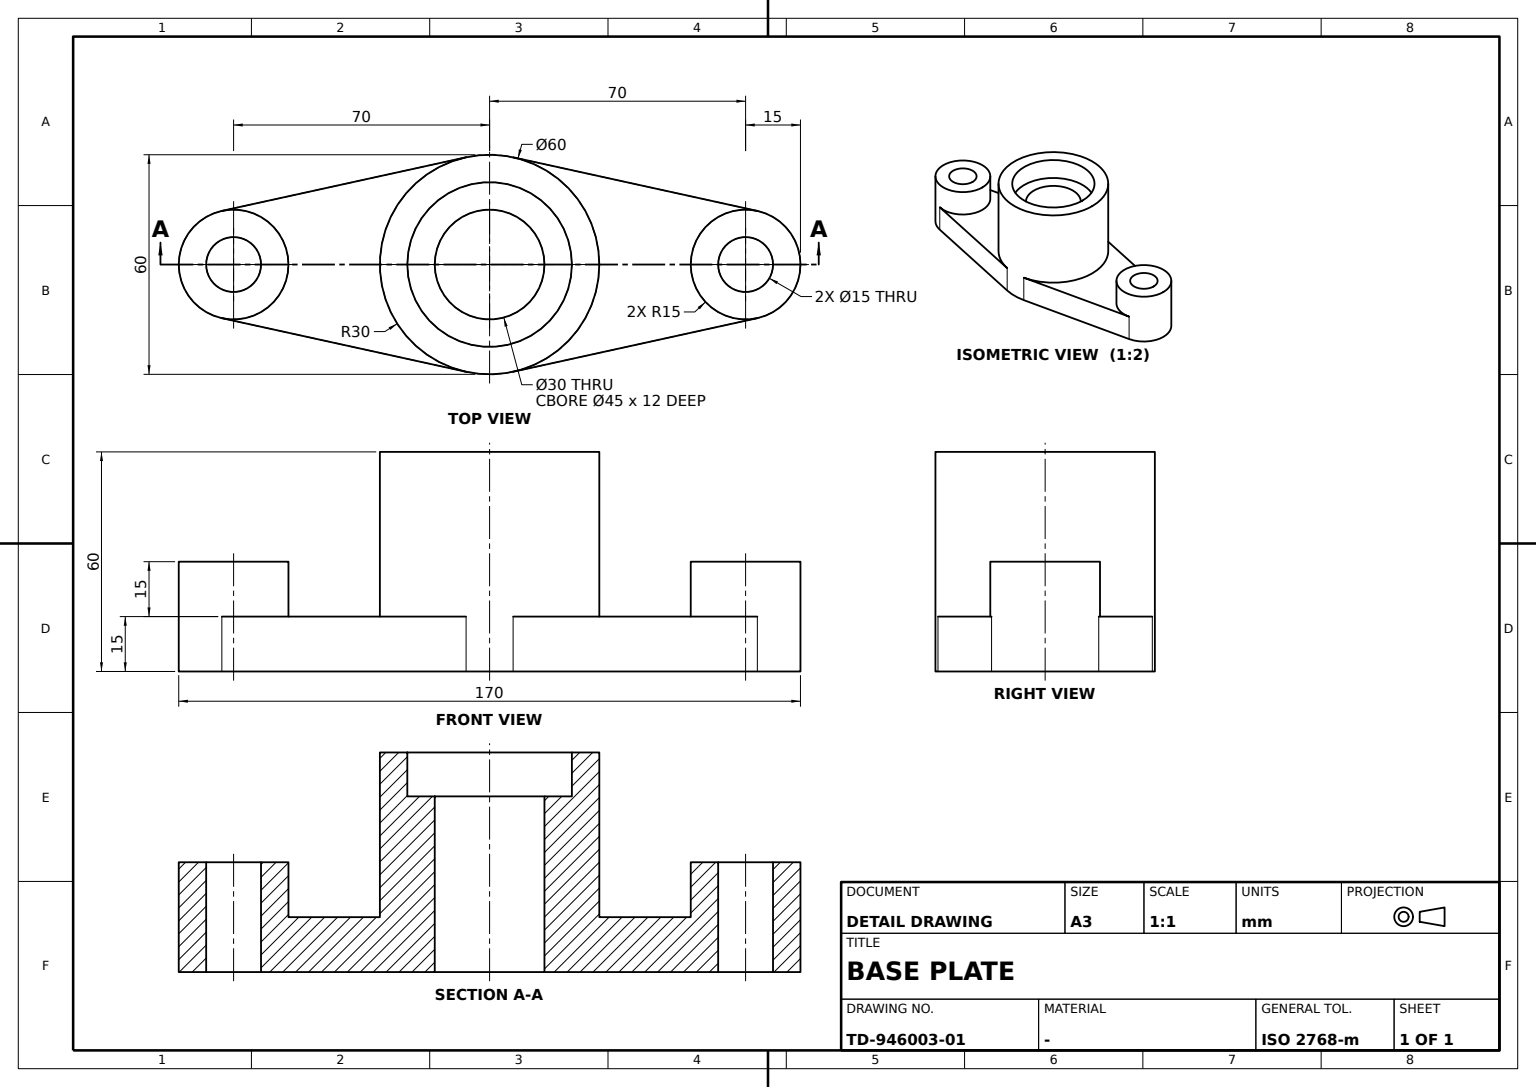
ISO-10303-21;
HEADER;
FILE_DESCRIPTION((''),'2;1');
FILE_NAME('','',(''),(''),'','','');
FILE_SCHEMA(('AUTOMOTIVE_DESIGN'));
ENDSEC;
DATA;
#1=APPLICATION_CONTEXT('');
#2=PRODUCT_CONTEXT('',#1,'mechanical');
#3=PRODUCT('','','',(#2));
#4=PRODUCT_DEFINITION_FORMATION('','',#3);
#5=PRODUCT_DEFINITION_CONTEXT('',#1,'design');
#6=PRODUCT_DEFINITION('','',#4,#5);
#7=PRODUCT_DEFINITION_SHAPE('','',#6);
#8=(LENGTH_UNIT()NAMED_UNIT(*)SI_UNIT(.MILLI.,.METRE.));
#9=(NAMED_UNIT(*)PLANE_ANGLE_UNIT()SI_UNIT($,.RADIAN.));
#10=(NAMED_UNIT(*)SI_UNIT($,.STERADIAN.)SOLID_ANGLE_UNIT());
#11=UNCERTAINTY_MEASURE_WITH_UNIT(LENGTH_MEASURE(0.005),#8,'distance_accuracy_value','');
#12=(GEOMETRIC_REPRESENTATION_CONTEXT(3)GLOBAL_UNCERTAINTY_ASSIGNED_CONTEXT((#11))GLOBAL_UNIT_ASSIGNED_CONTEXT((#8,#9,#10))REPRESENTATION_CONTEXT('',''));
#13=CARTESIAN_POINT('',(73.214286,14.651565,0.));
#14=VERTEX_POINT('',#13);
#15=CARTESIAN_POINT('',(73.214286,14.651565,15.));
#16=VERTEX_POINT('',#15);
#17=DIRECTION('',(0.,0.,1.));
#18=VECTOR('',#17,1000.);
#19=LINE('',#15,#18);
#20=EDGE_CURVE('',#14,#16,#19,.T.);
#21=ORIENTED_EDGE('',*,*,#20,.T.);
#22=CARTESIAN_POINT('',(73.214286,-14.651565,15.));
#23=VERTEX_POINT('',#22);
#24=CARTESIAN_POINT('',(70.,0.,15.));
#25=DIRECTION('',(1.,0.,0.));
#26=AXIS2_PLACEMENT_3D('',#24,#17,#25);
#27=CIRCLE('',#26,15.);
#28=EDGE_CURVE('',#16,#23,#27,.T.);
#29=ORIENTED_EDGE('',*,*,#28,.T.);
#30=CARTESIAN_POINT('',(73.214286,-14.651565,0.));
#31=VERTEX_POINT('',#30);
#32=LINE('',#22,#18);
#33=EDGE_CURVE('',#31,#23,#32,.T.);
#34=ORIENTED_EDGE('',*,*,#33,.F.);
#35=CARTESIAN_POINT('',(70.,0.,0.));
#36=AXIS2_PLACEMENT_3D('',#35,#17,#25);
#37=CIRCLE('',#36,15.);
#38=EDGE_CURVE('',#31,#14,#37,.T.);
#39=ORIENTED_EDGE('',*,*,#38,.T.);
#40=EDGE_LOOP('',(#21,#29,#34,#39));
#41=FACE_BOUND('',#40,.T.);
#42=CARTESIAN_POINT('',(85.,0.,30.));
#43=VERTEX_POINT('',#42);
#44=CARTESIAN_POINT('',(70.,0.,30.));
#45=AXIS2_PLACEMENT_3D('',#44,#17,#25);
#46=CIRCLE('',#45,15.);
#47=EDGE_CURVE('',#43,#43,#46,.T.);
#48=ORIENTED_EDGE('',*,*,#47,.F.);
#49=EDGE_LOOP('',(#48));
#50=FACE_BOUND('',#49,.T.);
#51=CYLINDRICAL_SURFACE('',#26,15.);
#52=ADVANCED_FACE('',(#41,#50),#51,.T.);
#53=CARTESIAN_POINT('',(-73.214286,-14.651565,15.));
#54=VERTEX_POINT('',#53);
#55=CARTESIAN_POINT('',(-6.428571,-29.303131,15.));
#56=VERTEX_POINT('',#55);
#57=DIRECTION('',(0.976771024,-0.214285714,0.));
#58=VECTOR('',#57,1000.);
#59=LINE('',#55,#58);
#60=EDGE_CURVE('',#54,#56,#59,.T.);
#61=ORIENTED_EDGE('',*,*,#60,.F.);
#62=CARTESIAN_POINT('',(-73.214286,-14.651565,0.));
#63=VERTEX_POINT('',#62);
#64=LINE('',#53,#18);
#65=EDGE_CURVE('',#63,#54,#64,.T.);
#66=ORIENTED_EDGE('',*,*,#65,.F.);
#67=CARTESIAN_POINT('',(-6.428571,-29.303131,0.));
#68=VERTEX_POINT('',#67);
#69=LINE('',#67,#58);
#70=EDGE_CURVE('',#63,#68,#69,.T.);
#71=ORIENTED_EDGE('',*,*,#70,.T.);
#72=CARTESIAN_POINT('',(-6.428571,-29.303131,30.));
#73=LINE('',#72,#18);
#74=EDGE_CURVE('',#68,#56,#73,.T.);
#75=ORIENTED_EDGE('',*,*,#74,.T.);
#76=EDGE_LOOP('',(#61,#66,#71,#75));
#77=FACE_BOUND('',#76,.T.);
#78=DIRECTION('',(-0.214285714,-0.976771024,0.));
#79=AXIS2_PLACEMENT_3D('',#62,#78,#57);
#80=PLANE('',#79);
#81=ADVANCED_FACE('',(#77),#80,.T.);
#82=CARTESIAN_POINT('',(22.5,0.,60.));
#83=VERTEX_POINT('',#82);
#84=CARTESIAN_POINT('',(0.,0.,60.));
#85=AXIS2_PLACEMENT_3D('',#84,#17,#25);
#86=CIRCLE('',#85,22.5);
#87=EDGE_CURVE('',#83,#83,#86,.T.);
#88=ORIENTED_EDGE('',*,*,#87,.F.);
#89=EDGE_LOOP('',(#88));
#90=FACE_BOUND('',#89,.T.);
#91=CARTESIAN_POINT('',(30.,0.,60.));
#92=VERTEX_POINT('',#91);
#93=CIRCLE('',#85,30.);
#94=EDGE_CURVE('',#92,#92,#93,.T.);
#95=ORIENTED_EDGE('',*,*,#94,.T.);
#96=EDGE_LOOP('',(#95));
#97=FACE_BOUND('',#96,.T.);
#98=PLANE('',#85);
#99=ADVANCED_FACE('',(#90,#97),#98,.T.);
#100=CARTESIAN_POINT('',(-73.214286,14.651565,15.));
#101=VERTEX_POINT('',#100);
#102=CARTESIAN_POINT('',(-6.428571,29.303131,15.));
#103=VERTEX_POINT('',#102);
#104=DIRECTION('',(0.976771024,0.214285714,0.));
#105=VECTOR('',#104,1000.);
#106=LINE('',#102,#105);
#107=EDGE_CURVE('',#101,#103,#106,.T.);
#108=ORIENTED_EDGE('',*,*,#107,.F.);
#109=CARTESIAN_POINT('',(-70.,0.,15.));
#110=AXIS2_PLACEMENT_3D('',#109,#17,#25);
#111=CIRCLE('',#110,15.);
#112=EDGE_CURVE('',#54,#101,#111,.T.);
#113=ORIENTED_EDGE('',*,*,#112,.F.);
#114=ORIENTED_EDGE('',*,*,#60,.T.);
#115=CARTESIAN_POINT('',(0.,0.,15.));
#116=AXIS2_PLACEMENT_3D('',#115,#17,#25);
#117=CIRCLE('',#116,30.);
#118=EDGE_CURVE('',#103,#56,#117,.T.);
#119=ORIENTED_EDGE('',*,*,#118,.F.);
#120=EDGE_LOOP('',(#108,#113,#114,#119));
#121=FACE_BOUND('',#120,.T.);
#122=PLANE('',#116);
#123=ADVANCED_FACE('',(#121),#122,.T.);
#124=ORIENTED_EDGE('',*,*,#87,.T.);
#125=EDGE_LOOP('',(#124));
#126=FACE_BOUND('',#125,.T.);
#127=CARTESIAN_POINT('',(22.5,0.,48.));
#128=VERTEX_POINT('',#127);
#129=CARTESIAN_POINT('',(0.,0.,48.));
#130=AXIS2_PLACEMENT_3D('',#129,#17,#25);
#131=CIRCLE('',#130,22.5);
#132=EDGE_CURVE('',#128,#128,#131,.T.);
#133=ORIENTED_EDGE('',*,*,#132,.F.);
#134=EDGE_LOOP('',(#133));
#135=FACE_BOUND('',#134,.T.);
#136=CARTESIAN_POINT('',(0.,0.,54.));
#137=AXIS2_PLACEMENT_3D('',#136,#17,#25);
#138=CYLINDRICAL_SURFACE('',#137,22.5);
#139=ADVANCED_FACE('',(#126,#135),#138,.F.);
#140=CARTESIAN_POINT('',(6.428571,29.303131,0.));
#141=VERTEX_POINT('',#140);
#142=CARTESIAN_POINT('',(6.428571,29.303131,15.));
#143=VERTEX_POINT('',#142);
#144=CARTESIAN_POINT('',(6.428571,29.303131,30.));
#145=LINE('',#144,#18);
#146=EDGE_CURVE('',#141,#143,#145,.T.);
#147=ORIENTED_EDGE('',*,*,#146,.T.);
#148=LINE('',#142,#58);
#149=EDGE_CURVE('',#143,#16,#148,.T.);
#150=ORIENTED_EDGE('',*,*,#149,.T.);
#151=ORIENTED_EDGE('',*,*,#20,.F.);
#152=LINE('',#140,#58);
#153=EDGE_CURVE('',#141,#14,#152,.T.);
#154=ORIENTED_EDGE('',*,*,#153,.F.);
#155=EDGE_LOOP('',(#147,#150,#151,#154));
#156=FACE_BOUND('',#155,.T.);
#157=AXIS2_PLACEMENT_3D('',#140,#78,#57);
#158=PLANE('',#157);
#159=ADVANCED_FACE('',(#156),#158,.F.);
#160=CARTESIAN_POINT('',(-62.5,0.,30.));
#161=VERTEX_POINT('',#160);
#162=CARTESIAN_POINT('',(-70.,0.,30.));
#163=AXIS2_PLACEMENT_3D('',#162,#17,#25);
#164=CIRCLE('',#163,7.5);
#165=EDGE_CURVE('',#161,#161,#164,.T.);
#166=ORIENTED_EDGE('',*,*,#165,.T.);
#167=EDGE_LOOP('',(#166));
#168=FACE_BOUND('',#167,.T.);
#169=CARTESIAN_POINT('',(-62.5,0.,0.));
#170=VERTEX_POINT('',#169);
#171=CARTESIAN_POINT('',(-70.,0.,0.));
#172=AXIS2_PLACEMENT_3D('',#171,#17,#25);
#173=CIRCLE('',#172,7.5);
#174=EDGE_CURVE('',#170,#170,#173,.T.);
#175=ORIENTED_EDGE('',*,*,#174,.F.);
#176=EDGE_LOOP('',(#175));
#177=FACE_BOUND('',#176,.T.);
#178=CYLINDRICAL_SURFACE('',#163,7.5);
#179=ADVANCED_FACE('',(#168,#177),#178,.F.);
#180=ORIENTED_EDGE('',*,*,#132,.T.);
#181=EDGE_LOOP('',(#180));
#182=FACE_BOUND('',#181,.T.);
#183=CARTESIAN_POINT('',(15.,0.,48.));
#184=VERTEX_POINT('',#183);
#185=CIRCLE('',#130,15.);
#186=EDGE_CURVE('',#184,#184,#185,.T.);
#187=ORIENTED_EDGE('',*,*,#186,.F.);
#188=EDGE_LOOP('',(#187));
#189=FACE_BOUND('',#188,.T.);
#190=PLANE('',#130);
#191=ADVANCED_FACE('',(#182,#189),#190,.T.);
#192=ORIENTED_EDGE('',*,*,#38,.F.);
#193=CARTESIAN_POINT('',(6.428571,-29.303131,0.));
#194=VERTEX_POINT('',#193);
#195=LINE('',#193,#105);
#196=EDGE_CURVE('',#194,#31,#195,.T.);
#197=ORIENTED_EDGE('',*,*,#196,.F.);
#198=CARTESIAN_POINT('',(0.,0.,0.));
#199=AXIS2_PLACEMENT_3D('',#198,#17,#25);
#200=CIRCLE('',#199,30.);
#201=EDGE_CURVE('',#68,#194,#200,.T.);
#202=ORIENTED_EDGE('',*,*,#201,.F.);
#203=ORIENTED_EDGE('',*,*,#70,.F.);
#204=CARTESIAN_POINT('',(-73.214286,14.651565,0.));
#205=VERTEX_POINT('',#204);
#206=CIRCLE('',#172,15.);
#207=EDGE_CURVE('',#205,#63,#206,.T.);
#208=ORIENTED_EDGE('',*,*,#207,.F.);
#209=CARTESIAN_POINT('',(-6.428571,29.303131,0.));
#210=VERTEX_POINT('',#209);
#211=LINE('',#209,#105);
#212=EDGE_CURVE('',#205,#210,#211,.T.);
#213=ORIENTED_EDGE('',*,*,#212,.T.);
#214=EDGE_CURVE('',#141,#210,#200,.T.);
#215=ORIENTED_EDGE('',*,*,#214,.F.);
#216=ORIENTED_EDGE('',*,*,#153,.T.);
#217=EDGE_LOOP('',(#192,#197,#202,#203,#208,#213,#215,#216));
#218=FACE_BOUND('',#217,.T.);
#219=CARTESIAN_POINT('',(15.,0.,0.));
#220=VERTEX_POINT('',#219);
#221=CIRCLE('',#199,15.);
#222=EDGE_CURVE('',#220,#220,#221,.T.);
#223=ORIENTED_EDGE('',*,*,#222,.T.);
#224=EDGE_LOOP('',(#223));
#225=FACE_BOUND('',#224,.T.);
#226=ORIENTED_EDGE('',*,*,#174,.T.);
#227=EDGE_LOOP('',(#226));
#228=FACE_BOUND('',#227,.T.);
#229=CARTESIAN_POINT('',(77.5,0.,0.));
#230=VERTEX_POINT('',#229);
#231=CIRCLE('',#36,7.5);
#232=EDGE_CURVE('',#230,#230,#231,.T.);
#233=ORIENTED_EDGE('',*,*,#232,.T.);
#234=EDGE_LOOP('',(#233));
#235=FACE_BOUND('',#234,.T.);
#236=PLANE('',#199);
#237=ADVANCED_FACE('',(#218,#225,#228,#235),#236,.F.);
#238=ORIENTED_EDGE('',*,*,#65,.T.);
#239=ORIENTED_EDGE('',*,*,#112,.T.);
#240=LINE('',#100,#18);
#241=EDGE_CURVE('',#205,#101,#240,.T.);
#242=ORIENTED_EDGE('',*,*,#241,.F.);
#243=ORIENTED_EDGE('',*,*,#207,.T.);
#244=EDGE_LOOP('',(#238,#239,#242,#243));
#245=FACE_BOUND('',#244,.T.);
#246=CARTESIAN_POINT('',(-55.,0.,30.));
#247=VERTEX_POINT('',#246);
#248=CIRCLE('',#163,15.);
#249=EDGE_CURVE('',#247,#247,#248,.T.);
#250=ORIENTED_EDGE('',*,*,#249,.F.);
#251=EDGE_LOOP('',(#250));
#252=FACE_BOUND('',#251,.T.);
#253=CYLINDRICAL_SURFACE('',#110,15.);
#254=ADVANCED_FACE('',(#245,#252),#253,.T.);
#255=ORIENTED_EDGE('',*,*,#222,.F.);
#256=EDGE_LOOP('',(#255));
#257=FACE_BOUND('',#256,.T.);
#258=ORIENTED_EDGE('',*,*,#186,.T.);
#259=EDGE_LOOP('',(#258));
#260=FACE_BOUND('',#259,.T.);
#261=CARTESIAN_POINT('',(0.,0.,30.));
#262=AXIS2_PLACEMENT_3D('',#261,#17,#25);
#263=CYLINDRICAL_SURFACE('',#262,15.);
#264=ADVANCED_FACE('',(#257,#260),#263,.F.);
#265=CARTESIAN_POINT('',(6.428571,-29.303131,15.));
#266=VERTEX_POINT('',#265);
#267=LINE('',#265,#105);
#268=EDGE_CURVE('',#266,#23,#267,.T.);
#269=ORIENTED_EDGE('',*,*,#268,.T.);
#270=ORIENTED_EDGE('',*,*,#28,.F.);
#271=ORIENTED_EDGE('',*,*,#149,.F.);
#272=EDGE_CURVE('',#266,#143,#117,.T.);
#273=ORIENTED_EDGE('',*,*,#272,.F.);
#274=EDGE_LOOP('',(#269,#270,#271,#273));
#275=FACE_BOUND('',#274,.T.);
#276=ADVANCED_FACE('',(#275),#122,.T.);
#277=CARTESIAN_POINT('',(77.5,0.,30.));
#278=VERTEX_POINT('',#277);
#279=CIRCLE('',#45,7.5);
#280=EDGE_CURVE('',#278,#278,#279,.T.);
#281=ORIENTED_EDGE('',*,*,#280,.F.);
#282=EDGE_LOOP('',(#281));
#283=FACE_BOUND('',#282,.T.);
#284=ORIENTED_EDGE('',*,*,#47,.T.);
#285=EDGE_LOOP('',(#284));
#286=FACE_BOUND('',#285,.T.);
#287=PLANE('',#262);
#288=ADVANCED_FACE('',(#283,#286),#287,.T.);
#289=CARTESIAN_POINT('',(6.428571,-29.303131,30.));
#290=LINE('',#289,#18);
#291=EDGE_CURVE('',#194,#266,#290,.T.);
#292=ORIENTED_EDGE('',*,*,#291,.F.);
#293=ORIENTED_EDGE('',*,*,#196,.T.);
#294=ORIENTED_EDGE('',*,*,#33,.T.);
#295=ORIENTED_EDGE('',*,*,#268,.F.);
#296=EDGE_LOOP('',(#292,#293,#294,#295));
#297=FACE_BOUND('',#296,.T.);
#298=DIRECTION('',(0.214285714,-0.976771024,0.));
#299=AXIS2_PLACEMENT_3D('',#193,#298,#104);
#300=PLANE('',#299);
#301=ADVANCED_FACE('',(#297),#300,.T.);
#302=ORIENTED_EDGE('',*,*,#249,.T.);
#303=EDGE_LOOP('',(#302));
#304=FACE_BOUND('',#303,.T.);
#305=ORIENTED_EDGE('',*,*,#165,.F.);
#306=EDGE_LOOP('',(#305));
#307=FACE_BOUND('',#306,.T.);
#308=ADVANCED_FACE('',(#304,#307),#287,.T.);
#309=ORIENTED_EDGE('',*,*,#232,.F.);
#310=EDGE_LOOP('',(#309));
#311=FACE_BOUND('',#310,.T.);
#312=ORIENTED_EDGE('',*,*,#280,.T.);
#313=EDGE_LOOP('',(#312));
#314=FACE_BOUND('',#313,.T.);
#315=CYLINDRICAL_SURFACE('',#45,7.5);
#316=ADVANCED_FACE('',(#311,#314),#315,.F.);
#317=CARTESIAN_POINT('',(-6.428571,29.303131,30.));
#318=LINE('',#317,#18);
#319=EDGE_CURVE('',#210,#103,#318,.T.);
#320=ORIENTED_EDGE('',*,*,#319,.F.);
#321=ORIENTED_EDGE('',*,*,#212,.F.);
#322=ORIENTED_EDGE('',*,*,#241,.T.);
#323=ORIENTED_EDGE('',*,*,#107,.T.);
#324=EDGE_LOOP('',(#320,#321,#322,#323));
#325=FACE_BOUND('',#324,.T.);
#326=AXIS2_PLACEMENT_3D('',#204,#298,#104);
#327=PLANE('',#326);
#328=ADVANCED_FACE('',(#325),#327,.F.);
#329=ORIENTED_EDGE('',*,*,#319,.T.);
#330=ORIENTED_EDGE('',*,*,#118,.T.);
#331=ORIENTED_EDGE('',*,*,#74,.F.);
#332=ORIENTED_EDGE('',*,*,#201,.T.);
#333=ORIENTED_EDGE('',*,*,#291,.T.);
#334=ORIENTED_EDGE('',*,*,#272,.T.);
#335=ORIENTED_EDGE('',*,*,#146,.F.);
#336=ORIENTED_EDGE('',*,*,#214,.T.);
#337=EDGE_LOOP('',(#329,#330,#331,#332,#333,#334,#335,#336));
#338=FACE_BOUND('',#337,.T.);
#339=ORIENTED_EDGE('',*,*,#94,.F.);
#340=EDGE_LOOP('',(#339));
#341=FACE_BOUND('',#340,.T.);
#342=CYLINDRICAL_SURFACE('',#262,30.);
#343=ADVANCED_FACE('',(#338,#341),#342,.T.);
#344=CLOSED_SHELL('',(#52,#81,#99,#123,#139,#159,#179,#191,#237,#254,#264,#276,#288,#301,#308,#316,#328,#343));
#345=MANIFOLD_SOLID_BREP('',#344);
#346=ADVANCED_BREP_SHAPE_REPRESENTATION('',(#345),#12);
#347=SHAPE_DEFINITION_REPRESENTATION(#7,#346);
ENDSEC;
END-ISO-10303-21;
